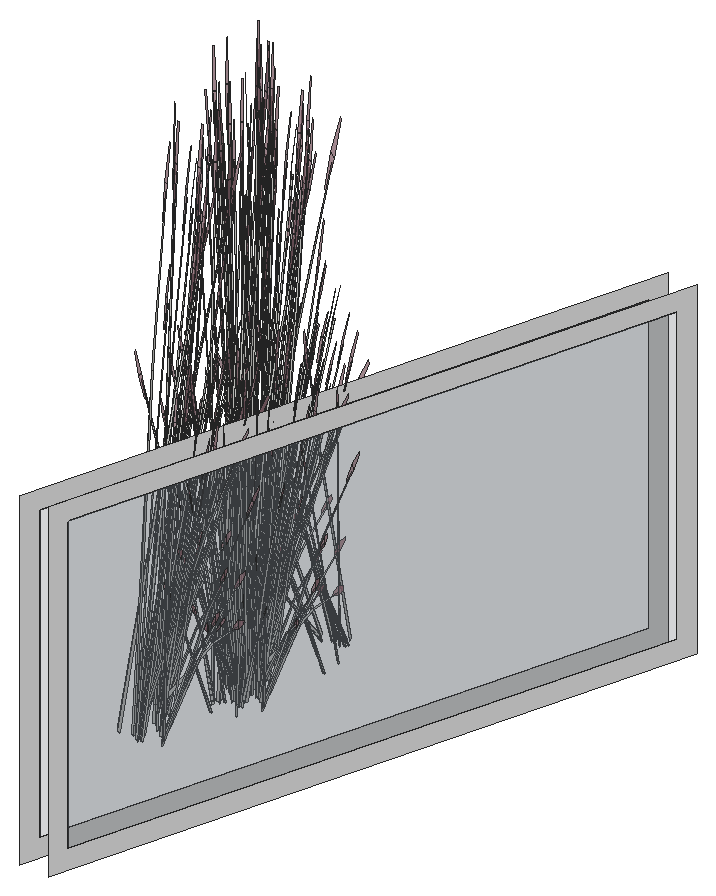
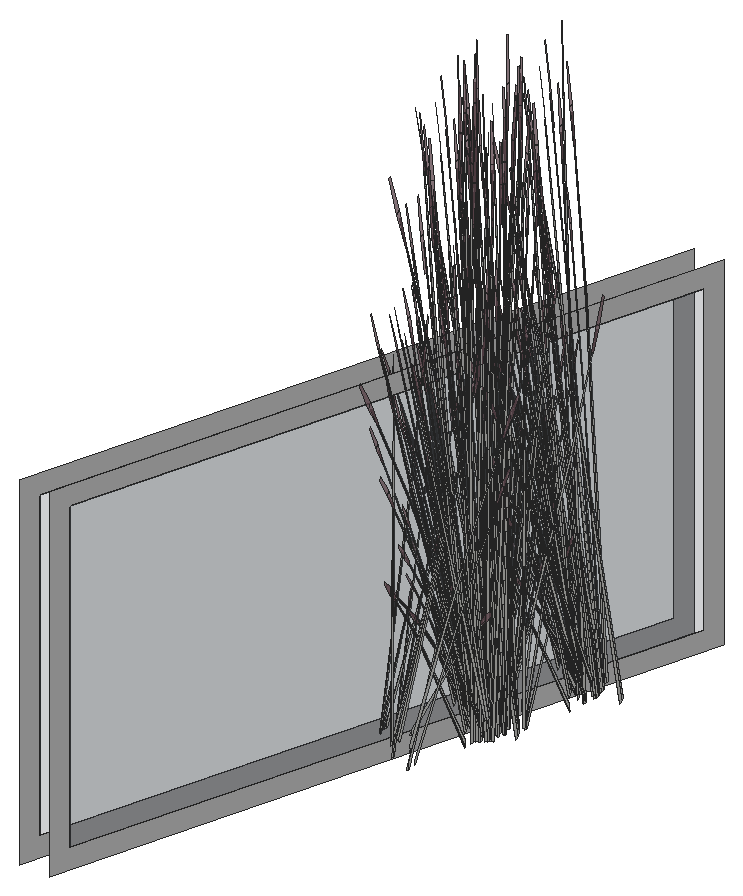
# SketchUp Ruby script. Lengths in inches.
U = 1.inch
M = Sketchup.active_model
def pt(a) = Geom::Point3d.new(a.map { |v| v * U })
def face(e, loops, mat)
  f = e.add_face(loops[0].map { |a| pt(a) })
  loops[1..].each { |l| e.add_face(l.map { |a| pt(a) }).erase! }
  f.material = f.back_material = mat if mat
  f
end
# faces: each face lists its corners as indices into pts; further lists are holes
def faces(e, pts, list, mat = nil) = list.each { |f| face(e, (f[0].is_a?(Array) ? f : [f]).map { |l| l.map { |i| pts[i] } }, mat) }
# xy, xz, yz: faces in a plane at the given z, y or x. An outline is a flat list of corners, or four numbers for a rectangle; further outlines are holes
def ring(l) = l.size == 4 ? [[l[0], l[1]], [l[2], l[1]], [l[2], l[3]], [l[0], l[3]]] : l.each_slice(2).to_a
def flat(e, list, mat, &to3) = list.each { |f| face(e, (f[0].is_a?(Array) ? f : [f]).map { |l| ring(l).map { |u, v| to3.(u, v) } }, mat) }
def xy(e, z, list, mat = nil) = flat(e, list, mat) { |x, y| [x, y, z] }
def xz(e, y, list, mat = nil) = flat(e, list, mat) { |x, z| [x, y, z] }
def yz(e, x, list, mat = nil) = flat(e, list, mat) { |y, z| [x, y, z] }
def lines(e, pts, list) = list.each { |a, b| e.add_line(pt(pts[a]), pt(pts[b])) }
# prism: a flat outline (further loops are holes) pulled along v
def prism(e, loops, v, mat = nil)
  f = face(e, loops, mat); d = Geom::Vector3d.new(v.map { |x| x * U })
  f.pushpull(f.normal.samedirection?(d) ? d.length : -d.length)
end
def box(e, o, s, mat = nil) = prism(e, [[o, [o[0] + s[0], o[1], o[2]], [o[0] + s[0], o[1] + s[1], o[2]], [o[0], o[1] + s[1], o[2]]]], [0, 0, s[2]], mat)
def at(x, y, z, deg = 0) = Geom::Transformation.translation(pt([x, y, z])) * Geom::Transformation.rotation(ORIGIN, Z_AXIS, deg.degrees)
def axes(o, x, y, z) = Geom::Transformation.new([*x, 0, *y, 0, *z, 0, *pt(o).to_a, 1])
def part(name) = M.definitions.add(name)
# library, detail: a bought-in or finely detailed component or shape, given as its bounding box
def library(name, o, s) = part(name).tap { |d| box(d.entities, o, s) }
def detail(e, o, s) = box(e.add_group.entities, o, s)
def put(e, d, t, mat = nil) = e.add_instance(d, t).tap { |i| i.material = mat if mat }
def group(e, t, mat = nil) = e.add_group.tap { |g| g.transformation = t; g.material = mat if mat }.entities
root = M.entities
M.materials.add("Glass_Basic_01").color = [105, 113, 122]
M.materials["Glass_Basic_01"].alpha = 0.25
M.materials.add("LightPink_Translucent").color = [144, 107, 117]
M.materials["LightPink_Translucent"].alpha = 0.75
M.materials.add("M01_Silver_Fog").color = [224, 224, 224]
c1 = part("blade")
p = [[2.15,0.21,22],[0,0.17,0],[0.09,0.45,0],[2.18,0.31,22],[2.29,0.31,22],[0.38,0.45,0],
  [2.48,0.24,33],[2.49,0.24,33],[2.48,0.22,33]]
faces(c1.entities,p,[[0,1,2,3],[4,5,2,3],[6,3,4,7],[8,0,3,6]])
c2 = part("seeds")
p = [[0.3,-0.1,1.38],[-0.01,-0.03,1.59],[-0.01,-0.03,0.03],[0.14,-0.07,-0.07],[0.29,-0.03,3],[0.15,0.01,3.11]]
faces(c2.entities,p,[[0,1,2,3],[1,0,4,5]],"LightPink_Translucent")
c3 = part("blade with seeds")
put(c3.entities,c1,at(0,0,0))
put(c3.entities,c2,axes([2.4,0.25,30.99],[1.5799,-0.05474,1.17369],[-0.12525,1.92788,0.29478],[-0.07173,-0.02425,1.56792]))
p = [[321.22,307.35,306],[340.07,371.78,306],[340.07,371.78,270],[321.22,307.35,270],[339.51,369.86,272],[339.51,369.86,304],
  [321.78,309.27,304],[321.78,309.27,272],[343.2,371.78,306],[324.34,307.35,306],[324.34,307.35,270],[343.2,371.78,270],
  [324.9,309.27,272],[324.9,309.27,304],[342.64,369.86,304],[342.64,369.86,272]]
faces(root,p,[[[0,1,2,3],[4,5,6,7]],[[8,9,10,11],[12,13,14,15]]],"M01_Silver_Fog")
faces(root,p,[[5,4,7,6],[13,12,15,14]],"Glass_Basic_01")
put(root,c3,axes([321.23,333.72,274.13],[-0.34721,0.30895,-0.03893],[-0.31814,-0.33837,-0.17649],[-0.0224,-0.09588,0.58215]))
put(root,c3,axes([321.09,336.77,274.36],[0.63506,0.11347,0.45755],[-0.12924,0.64083,0.17955],[-0.09281,-0.06188,1.58856]))
put(root,c3,axes([319.37,326.4,274.67],[0.56585,0.25696,-0.29095],[-0.27246,0.54236,-0.50002],[0.01778,0.13316,1.59708]))
put(root,c3,axes([320.92,336.65,274.72],[-0.24378,0.48527,0.44739],[-0.50654,-0.23354,-0.21531],[0,-0.11186,1.43643]))
put(root,c3,axes([321.73,334.32,276.98],[-0.23981,-0.43789,-0.71045],[0.49365,-0.24404,0.08574],[-0.05608,-0.21158,1.00501]))
put(root,c3,axes([320.75,337.79,274.47],[0.53992,-0.14294,0.17642],[0.13332,0.53195,0.35086],[-0.04815,-0.07751,1.60407]))
put(root,c3,axes([320.6,326.53,274.48],[0,-0.53854,0.49651],[0.56215,0,0],[0,0.12266,1.57504]))
put(root,c3,axes([320.84,327.03,274.02],[0,0.53854,-0.49651],[-0.56215,0,0],[0,0.12266,1.57504]))
put(root,c3,axes([319.34,328.66,276.73],[-0.49974,0.12359,0.48003],[-0.08673,-0.48481,0.3958],[0.11753,0.14288,0.9933]))
put(root,c3,axes([319.24,328.75,276.73],[-0.22836,0.34211,0.0643],[-0.3252,-0.19918,0.50621],[0.10513,0.10968,0.77189]))
put(root,c3,axes([321.44,337.88,274.2],[-0.50654,-0.24178,0],[0.24378,-0.50239,0],[0,0,1.62707]))
put(root,c3,axes([321.82,334.38,277.05],[-0.15148,0.41415,0.35414],[-0.44193,-0.12079,-0.4572],[-0.04052,-0.16674,0.87481]))
put(root,c3,axes([318.66,327.625,275.875],[-0.11485,-0.17291,1.71376],[0.53072,-0.14557,0.13857],[0.11995,0.27145,0.73262]))
put(root,c3,axes([322.61,338.48,274.375],[0.31414,0.53965,0],[-0.52557,0.30095,-0.51607],[-0.1197,0.06854,1.63711]))
put(root,c3,axes([319,325.68,274.62],[0.09693,-0.48062,0.1448],[0.47357,0.08343,-0.41347],[0.08619,0.04935,1.26744]))
put(root,c3,axes([321.02,338.72,277.0625],[-0.4951,-0.14079,0.53283],[0.1693,-0.46287,0.43934],[0.02975,0.18203,1.10256]))
put(root,c3,axes([320.88,338.75,276.73],[-0.37023,0.18303,0.0643],[-0.18122,-0.33376,0.50621],[0.03575,0.14712,0.77189]))
put(root,c3,axes([319.67,324.84,274.48],[-0.47024,-0.26927,0.49651],[0.28107,-0.48284,0],[0.1071,0.06133,1.57504]))
put(root,c3,axes([322.35,337.82,274.47],[0.14515,-0.53522,0.17642],[0.53115,0.15146,0.35086],[-0.09175,0.00261,1.60407]))
put(root,c3,axes([322.11,337.11,274.62],[0.37121,0.32357,0.1448],[-0.30963,0.36505,-0.41347],[-0.08619,0.04935,1.26744]))
put(root,c3,axes([321.98,336.71,274.3],[-0.46736,-0.46353,-0.06131],[0.46764,-0.46381,0],[-0.01632,-0.01619,1.75571]))
put(root,c3,axes([319.26,327.66,274.18],[0.5275,-0.18273,-0.19198],[0.18536,0.52636,0.00008],[0.05823,-0.0202,1.73897]))
put(root,c3,axes([322.1,336.875,274.72],[0.54562,-0.03324,0.44739],[0.04934,0.55185,-0.21531],[-0.09768,0.05593,1.43643]))
put(root,c3,axes([322.23,338.15,274.33],[0.62903,0.17504,0.30756],[-0.15737,0.62568,-0.36492],[-0.10411,0.07831,1.64885]))
put(root,c3,axes([321.31,333.35,273.49],[-0.08428,0.0194,1.76342],[-0.46606,-0.21841,-0.26939],[0.00782,-0.18218,0.30037]))
put(root,c3,axes([322.5,338.11,274.48],[0.47024,-0.26927,0.49651],[0.28107,0.48284,0],[-0.1071,0.06133,1.57504]))
put(root,c3,axes([319.17,328.36,277.05],[-0.0776,-0.43378,0.35414],[0.44361,-0.11454,-0.4572],[0.11915,0.12431,0.87481]))
put(root,c3,axes([321.77,333.94,276.53],[0.15148,-0.41415,-0.35414],[0.44193,0.12079,0.4572],[-0.04052,-0.16674,0.87481]))
put(root,c3,axes([321.03,336.18,274.36],[0.21845,0.6022,0.45755],[-0.62418,0.20941,0.17955],[0.00763,-0.11065,1.58856]))
put(root,c3,axes([319.27,326.09,274.21],[0.30184,0.45202,-0.44739],[-0.45719,0.31831,0.21531],[0.09768,0.05593,1.43643]))
put(root,c3,axes([320.93,336.1,274.21],[0.24378,-0.48527,-0.44739],[0.50654,0.23354,0.21531],[0,-0.11186,1.43643]))
put(root,c3,axes([321.56,337.67,274.2],[-0.16394,-0.4643,0],[0.46814,-0.1626,0],[0,0,1.54371]))
put(root,c3,axes([323.47,345,274.59],[-0.03043,0.17617,1.43002],[-0.4448,0.14748,-0.30754],[-0.10397,-0.22771,0.61141]))
put(root,c3,axes([319.47,325.87,276.47],[-0.43417,-0.27982,1.38283],[0.45844,-0.43566,0.59665],[0.14008,0.26255,1.33663]))
put(root,c3,axes([323.61,345.46,275.875],[0.11485,0.17291,1.71376],[-0.53072,0.14557,0.13857],[-0.11995,-0.27145,0.73262]))
put(root,c3,axes([318.74,328.97,276.71],[0.00149,-0.0652,1.77383],[0.43058,-0.28766,-0.16761],[0.14956,0.10267,0.31391]))
put(root,c3,axes([320.125,328.14,274.77],[-0.2829,-0.15485,1.1486],[0.36529,-0.15734,0.84392],[0.09853,0.13328,0.25299]))
put(root,c3,axes([319.12,327.98,274.59],[0.00887,-0.17852,1.43002],[0.42372,-0.19941,-0.30754],[0.1308,0.21367,0.61141]))
put(root,c3,axes([322.22,336.75,274.21],[-0.24378,0.48527,-0.44739],[-0.50654,-0.23354,0.21531],[0,0.11186,1.43643]))
put(root,c3,axes([320.1,325.09,274.03],[0.11803,0.46926,-0.30978],[-0.46876,0.13325,0.30978],[0.0945,0.05411,1.38974]))
put(root,c3,axes([321.96,334.01,276.73],[0.37023,-0.18303,0.0643],[0.18122,0.33376,0.50621],[-0.03575,-0.14712,0.77189]))
put(root,c3,axes([320.98,326.62,274.375],[0.62828,0,0],[0,0.6019,-0.51607],[0,0.13709,1.63711]))
put(root,c3,axes([323.18,336.46,274.47],[-0.39477,-0.39228,0.17642],[0.39783,-0.38049,0.35086],[-0.0436,0.08011,1.60407]))
put(root,c3,axes([321.82,336.23,274.21],[0,-0.62313,0],[0.62828,0,0],[0,0,1.79456]))
put(root,c3,axes([321.83,334.04,276.73],[0.4951,0.14079,0.48003],[-0.1693,0.46287,0.3958],[-0.02975,-0.18203,0.9933]))
put(root,c3,axes([321.24,336.35,274.43],[0.56613,0.26102,0.24065],[-0.27246,0.54236,0.50002],[0,-0.12502,1.60543]))
put(root,c3,axes([322.14,336.48,274.29],[0,0.62282,-0.05637],[-0.62828,0,0],[0,0.01957,1.79368]))
put(root,c3,axes([318.95,325.84,274.67],[0.5073,-0.35754,-0.29095],[0.33735,0.5052,-0.50002],[0.12516,0.05131,1.59708]))
put(root,c3,axes([321.05,335.98,274.72],[-0.54562,0.03324,0.44739],[-0.04934,-0.55185,-0.21531],[0.09768,-0.05593,1.43643]))
put(root,c3,axes([320.17,328.85,274.67],[-0.3222,-0.01689,1.0506],[0.21278,-0.35872,0.58006],[0.12729,0.12745,0.8241]))
put(root,c3,axes([321.02,338.375,277.05],[0.15148,-0.41415,0.35414],[0.44193,0.12079,-0.4572],[0.04052,0.16674,0.87481]))
put(root,c3,axes([320.8,335.03,274.47],[-0.14515,0.53522,0.17642],[-0.53115,-0.15146,0.35086],[0.09175,-0.00261,1.60407]))
put(root,c3,axes([321.83,337.69,274.29],[0.21845,0.61869,-0.06012],[-0.62418,0.21679,0],[0.00763,0.02161,1.72173]))
put(root,c3,axes([320.54,334.375,274.375],[-0.31414,-0.53965,0],[0.52557,-0.30095,-0.51607],[0.1197,-0.06854,1.63711]))
put(root,c3,axes([323.64,336.875,274.2],[-0.62797,-0.00431,-0.04976],[0,-0.6019,0.49943],[-0.01973,0.13702,1.58352]))
put(root,c3,axes([319.13,328.59,277.03],[0.2994,-0.46097,-0.1216],[0.43359,0.26557,-0.67495],[0.15072,0.13024,1.02557]))
put(root,c3,axes([317.67,325.52,273.59],[-0.49456,0.21561,1.28929],[-0.15741,-0.61865,0.50096],[0.30369,0.01029,1.46642]))
put(root,c3,axes([322.41,335.0625,274.47],[-0.53992,0.14294,0.17642],[-0.13332,-0.53195,0.35086],[0.04815,0.07751,1.60407]))
put(root,c3,axes([321.85,333.07,274.77],[0.06446,0.31404,1.1486],[-0.35756,-0.17393,0.84392],[0.03848,-0.1608,0.25299]))
put(root,c3,axes([321.62,339.85,277.65],[0.34721,-0.30895,-0.06488],[0.31814,0.33837,-0.29416],[0.0224,0.09588,0.97024]))
put(root,c3,axes([319.49,328.36,276.68],[0.4958,-0.12802,-0.51099],[0.08673,0.48481,-0.3958],[0.13317,0.13893,0.97773]))
put(root,c3,axes([321.52,335.84,274.36],[-0.4166,0.48873,0.45755],[-0.49494,-0.43142,0.17955],[0.10044,-0.04877,1.58856]))
put(root,c3,axes([322.23,336.61,274.21],[0.35073,0.34786,0],[-0.35073,0.34786,0],[0,0,1.69266]))
put(root,c3,axes([319.94,324.5625,274.375],[0.31414,-0.53965,0],[0.52557,0.30095,-0.51607],[0.1197,0.06854,1.63711]))
put(root,c3,axes([322.23,336.2,274.72],[0.24378,-0.48527,0.44739],[0.50654,0.23354,-0.21531],[0,0.11186,1.43643]))
put(root,c3,axes([322.02,337.89,274.2],[0.50654,0.24178,0],[-0.24378,0.50239,0],[0,0,1.74954]))
put(root,c3,axes([320.05,327.77,277.05],[-0.28589,-0.33718,0.35414],[0.32644,-0.31919,-0.4572],[0.16586,0.04856,0.87481]))
put(root,c3,axes([320.23,324.89,274.02],[0.47024,0.26927,-0.49651],[-0.28107,0.48284,0],[0.1071,0.06133,1.57504]))
put(root,c3,axes([324.49,344.3125,276.72],[-0.07685,-0.07551,1.74944],[-0.51287,0.04787,-0.27667],[-0.08185,-0.1806,0.14031]))
put(root,c3,axes([320.875,338.55,277.03],[0.49168,-0.25073,-0.1216],[0.24162,0.44501,-0.67495],[0.06487,0.18753,1.02557]))
put(root,c3,axes([320.3125,328.08,276.73],[-0.0253,0.40952,0.0643],[-0.38204,-0.01123,0.50621],[0.14634,0.04285,0.77189]))
put(root,c3,axes([322.0625,336.09,274.38],[-0.63506,-0.11347,0.49198],[0.12924,-0.64083,0.19306],[0.09281,0.06188,1.70813]))
put(root,c3,axes([323.39,333.58,276.71],[-0.05103,0.04113,1.77383],[-0.49994,-0.13878,-0.16761],[-0.0181,-0.17951,0.31391]))
put(root,c3,axes([320.2,328.72,273.49],[0.03661,-0.07775,1.76342],[0.46087,-0.22898,-0.26939],[0.13972,0.11851,0.30037]))
put(root,c3,axes([322.99,334.77,277.03],[-0.55221,-0.02668,-0.1216],[0.01509,-0.50521,-0.67495],[0.03836,-0.19458,1.02557]))
put(root,c3,axes([320.35,327.95,276.73],[-0.37048,0.35486,0.48003],[-0.31952,-0.37685,0.3958],[0.17382,0.06546,0.9933]))
put(root,c3,axes([323.51,336.96,274.03],[-0.35073,0.33601,-0.30978],[-0.35073,-0.33601,0.30978],[0,0.10823,1.38974]))
put(root,c3,axes([321.3125,328,275.93],[-0.09617,-0.45271,-0.03492],[0.45453,-0.10408,-0.15832],[0.09492,0.0287,0.52218]))
put(root,c3,axes([320.52,326.83,277.05],[-0.41757,-0.15024,0.35414],[0.12179,-0.4383,-0.4572],[0.16812,-0.04019,0.87481]))
put(root,c3,axes([322.51,336.9,274.09],[0.18424,0.49308,-0.69212],[-0.53071,0.17758,-0.18165],[0.02036,0.16697,1.52773]))
put(root,c3,axes([322.25,336.37,274.21],[0.56215,0,0],[0,0.55754,0],[0,0,1.78407]))
put(root,c3,axes([319.54,325.92,274.06],[0.52267,0.08829,-0.62353],[-0.11029,0.54463,-0.16365],[0.15598,0.06599,1.37633]))
put(root,c3,axes([322.78,334.85,277.05],[-0.33997,0.28354,0.35414],[-0.32182,-0.32376,-0.4572],[0.04897,-0.1645,0.87481]))
put(root,c3,axes([321.71,335.76,274.72],[-0.30184,-0.45202,0.44739],[0.45719,-0.31831,-0.21531],[0.09768,0.05593,1.43643]))
put(root,c3,axes([321.77,326.24,274.26],[-0.31151,-0.34437,-0.06488],[0.34117,-0.31553,-0.29416],[0.09667,-0.02221,0.97024]))
put(root,c3,axes([321.16,335.86,274.67],[-0.05855,-0.61451,-0.29095],[0.60981,-0.03716,-0.50002],[0.10738,-0.08185,1.59708]))
put(root,c3,axes([322.44,336.3125,274.62],[0.46814,-0.15705,0.1448],[0.16394,0.44848,-0.41347],[0,0.0987,1.26744]))
put(root,c3,axes([322.62,334.58,276.68],[-0.35968,-0.36185,-0.51099],[0.37996,-0.3169,-0.3958],[0.05473,-0.18385,0.97773]))
put(root,c3,axes([324.85,345.5,276.68],[-0.49392,-0.135,-0.51099],[0.1693,-0.46287,-0.3958],[-0.04529,-0.18636,0.97773]))
put(root,c3,axes([322.28,336.35,274.67],[0.56585,0.25696,-0.29095],[-0.27246,0.54236,-0.50002],[0.01778,0.13316,1.59708]))
put(root,c3,axes([321.08,334.5,274.03],[0.46876,0.13325,-0.30978],[-0.11803,0.46926,0.30978],[0.0945,-0.05411,1.38974]))
put(root,c3,axes([322.38,333.9375,274.59],[-0.14282,0.10901,1.43002],[-0.42773,-0.19079,-0.30754],[0.07929,-0.23728,0.61141]))
put(root,c3,axes([319.43,327.09,275.875],[-0.18664,-0.09279,1.71376],[0.38624,-0.38925,0.13857],[0.24072,0.1756,0.73262]))
put(root,c3,axes([323.51,336.47,274.48],[0,-0.53854,0.49651],[0.56215,0,0],[0,0.12266,1.57504]))
put(root,c3,axes([323.75,336.97,274.02],[0,0.53854,-0.49651],[-0.56215,0,0],[0,0.12266,1.57504]))
put(root,c3,axes([322.25,338.6,276.73],[-0.49974,0.12359,0.48003],[-0.08673,-0.48481,0.3958],[0.11753,0.14288,0.9933]))
put(root,c3,axes([320.97,334.29,274.02],[0.47024,-0.26927,-0.49651],[0.28107,0.48284,0],[0.1071,-0.06133,1.57504]))
put(root,c3,axes([322.15,338.7,276.73],[-0.22836,0.34211,0.0643],[-0.3252,-0.19918,0.50621],[0.10513,0.10968,0.77189]))
put(root,c3,axes([321.91,335.63,274.62],[0.09693,-0.48062,0.1448],[0.47357,0.08343,-0.41347],[0.08619,0.04935,1.26744]))
put(root,c3,axes([325.03,345.59,276.98],[-0.23981,-0.43789,-0.71045],[0.49365,-0.24404,0.08574],[-0.05608,-0.21158,1.00501]))
put(root,c3,axes([320.9,326.97,276.73],[0.18454,0.3672,0.0643],[-0.33652,0.17973,0.50621],[0.14834,-0.03546,0.77189]))
put(root,c3,axes([320.46,327.95,276.53],[0.28589,0.33718,-0.35414],[-0.32644,0.31919,0.4572],[0.16586,0.04856,0.87481]))
put(root,c3,axes([320.13,327.99,277.03],[0.0269,-0.54769,-0.1216],[0.50939,0.01497,-0.67495],[0.19618,0.03804,1.02557]))
put(root,c3,axes([320.7,326.98,277.03],[-0.25281,-0.48765,-0.1216],[0.44869,-0.23964,-0.67495],[0.18908,-0.06434,1.02557]))
put(root,c3,axes([320.87,326.84,276.73],[-0.14195,0.49104,0.48003],[-0.46669,-0.16791,0.3958],[0.18353,-0.02951,0.9933]))
put(root,c3,axes([322.58,334.79,274.48],[-0.47024,-0.26927,0.49651],[0.28107,-0.48284,0],[0.1071,0.06133,1.57504]))
put(root,c3,axes([322.73,334.74,276.98],[0.01307,-0.49815,-0.71045],[0.55054,0.03346,0.08574],[0.0581,-0.21104,1.00501]))
put(root,c3,axes([322.17,337.6,274.18],[0.5275,-0.18273,-0.19198],[0.18536,0.52636,0.00008],[0.05823,-0.0202,1.73897]))
put(root,c3,axes([322.08,338.31,277.05],[-0.0776,-0.43378,0.35414],[0.44361,-0.11454,-0.4572],[0.11915,0.12431,0.87481]))
put(root,c3,axes([320.58,327.66,276.72],[0.10779,-0.00911,1.74944],[0.29564,-0.41839,-0.27667],[0.19172,0.05523,0.14031]))
put(root,c3,axes([322.18,336.04,274.21],[0.30184,0.45202,-0.44739],[-0.45719,0.31831,0.21531],[0.09768,0.05593,1.43643]))
put(root,c3,axes([320.68,326.56,276.68],[0.13612,-0.48987,-0.51099],[0.46669,0.16791,-0.3958],[0.1879,-0.04492,0.97773]))
put(root,c3,axes([322.38,335.8125,276.47],[-0.43417,-0.27982,1.38283],[0.45844,-0.43566,0.59665],[0.14008,0.26255,1.33663]))
put(root,c3,axes([322.95,334.45,276.53],[0.33997,-0.28354,-0.35414],[0.32182,0.32376,0.4572],[0.04897,-0.1645,0.87481]))
put(root,c3,axes([321.85,326.87,274.77],[-0.31044,0.08891,1.1486],[0.14613,-0.36744,0.84392],[0.16469,0.02514,0.25299]))
put(root,c3,axes([321.65,338.91,276.71],[0.00149,-0.0652,1.77383],[0.43058,-0.28766,-0.16761],[0.14956,0.10267,0.31391]))
put(root,c3,axes([323.08,334.59,276.73],[0.4129,0.02509,0.0643],[-0.01132,0.37891,0.50621],[0.04321,-0.14514,0.77189]))
put(root,c3,axes([323.04,338.09,274.77],[-0.2829,-0.15485,1.1486],[0.36529,-0.15734,0.84392],[0.09853,0.13328,0.25299]))
put(root,c3,axes([322.03,337.93,274.59],[0.00887,-0.17852,1.43002],[0.42372,-0.19941,-0.30754],[0.1308,0.21367,0.61141]))
put(root,c3,axes([324.61,344.62,273.49],[-0.08428,0.0194,1.76342],[-0.46606,-0.21841,-0.26939],[0.00782,-0.18218,0.30037]))
put(root,c3,axes([323.49,333.97,276.72],[-0.00485,-0.10718,1.74944],[-0.40965,-0.30977,-0.27667],[0.06333,-0.18778,0.14031]))
put(root,c3,axes([321.52,335.39,274.06],[0.33843,-0.40479,-0.62353],[0.42041,0.36705,-0.16365],[0.13561,-0.10098,1.37633]))
put(root,c3,axes([322.95,334.56,276.73],[0.35779,0.36745,0.48003],[-0.37996,0.3169,0.3958],[0.066,-0.17239,0.9933]))
put(root,c3,axes([320.96,326.78,276.53],[0.41757,0.15024,-0.35414],[-0.12179,0.4383,0.4572],[0.16812,-0.04019,0.87481]))
put(root,c3,axes([325.07,345.22,276.53],[0.15148,-0.41415,-0.35414],[0.44193,0.12079,0.4572],[-0.04052,-0.16674,0.87481]))
put(root,c3,axes([320.16,327.73,276.98],[0.50227,0.01297,-0.71045],[-0.03373,0.54602,0.08574],[0.21278,0.05762,1.00501]))
put(root,c3,axes([323.01,335.04,274.03],[0.11803,0.46926,-0.30978],[-0.46876,0.13325,0.30978],[0.0945,0.05411,1.38974]))
put(root,c3,axes([323.89,336.56,274.375],[0.62828,0,0],[0,0.6019,-0.51607],[0,0.13709,1.63711]))
put(root,c3,axes([321.18,326.7,273.98],[-0.32361,0.06463,1.41583],[-0.05151,-0.51444,0.08104],[0.22666,-0.07786,0.80566]))
put(root,c3,axes([321.53,326.36,273.49],[-0.02626,-0.08176,1.76342],[0.18213,-0.47826,-0.26939],[0.18372,-0.00688,0.30037]))
put(root,c3,axes([321.71,328.42,276.71],[-0.04543,-0.04715,1.77383],[0.09938,-0.50538,-0.16761],[0.17896,-0.03229,0.31391]))
put(root,c3,axes([321.86,335.78,274.67],[0.5073,-0.35754,-0.29095],[0.33735,0.5052,-0.50002],[0.12516,0.05131,1.59708]))
put(root,c3,axes([319.83,326.24,275.875],[-0.20841,0.0122,1.71376],[0.13825,-0.52864,0.13857],[0.297,0.0327,0.73262]))
put(root,c3,axes([323.08,338.8,274.67],[-0.3222,-0.01689,1.0506],[0.21278,-0.35872,0.58006],[0.12729,0.12745,0.8241]))
put(root,c3,axes([323.37,335.72,277.05],[-0.43736,0.07697,0.35414],[-0.11549,-0.43998,-0.4572],[0.12533,-0.11818,0.87481]))
put(root,c3,axes([322.11,334.49,275.875],[-0.09355,0.18511,1.71376],[-0.39247,-0.38307,0.13857],[0.17705,-0.23875,0.73262]))
put(root,c3,axes([320.59,326.74,276.98],[0.44151,-0.23785,-0.71045],[0.24605,0.4896,0.08574],[0.21333,-0.05562,1.00501]))
put(root,c3,axes([322.04,338.53,277.03],[0.2994,-0.46097,-0.1216],[0.43359,0.26557,-0.67495],[0.15072,0.13024,1.02557]))
put(root,c3,axes([320.58,335.47,273.59],[-0.49456,0.21561,1.28929],[-0.15741,-0.61865,0.50096],[0.30369,0.01029,1.46642]))
put(root,c3,axes([323.59,335.76,277.03],[-0.46478,-0.29695,-0.1216],[0.26776,-0.43004,-0.67495],[0.13131,-0.14949,1.02557]))
put(root,c3,axes([322.4,338.3,276.68],[0.4958,-0.12802,-0.51099],[0.08673,0.48481,-0.3958],[0.13317,0.13893,0.97773]))
put(root,c3,axes([321.27,327.46,274.59],[-0.12101,-0.13245,1.43002],[0.15744,-0.43816,-0.30754],[0.24483,0.05936,0.61141]))
put(root,c3,axes([322.85,334.51,274.375],[0.31414,-0.53965,0],[0.52557,0.30095,-0.51607],[0.1197,0.06854,1.63711]))
put(root,c3,axes([323.38,334.27,273.49],[-0.0752,-0.04243,1.76342],[-0.19317,-0.47398,-0.26939],[0.13031,-0.12863,0.30037]))
put(root,c3,axes([322.97,337.72,277.05],[-0.28589,-0.33718,0.35414],[0.32644,-0.31919,-0.4572],[0.16586,0.04856,0.87481]))
put(root,c3,axes([323.14,334.83,274.02],[0.47024,0.26927,-0.49651],[-0.28107,0.48284,0],[0.1071,0.06133,1.57504]))
put(root,c3,axes([323.23,338.03,276.73],[-0.0253,0.40952,0.0643],[-0.38204,-0.01123,0.50621],[0.14634,0.04285,0.77189]))
put(root,c3,axes([323.11,338.67,273.49],[0.03661,-0.07775,1.76342],[0.46087,-0.22898,-0.26939],[0.13972,0.11851,0.30037]))
put(root,c3,axes([323.26,337.9,276.73],[-0.37048,0.35486,0.48003],[-0.31952,-0.37685,0.3958],[0.17382,0.06546,0.9933]))
put(root,c3,axes([323.36,335.41,276.68],[-0.12908,-0.49174,-0.51099],[0.48882,-0.08602,-0.3958],[0.14008,-0.13208,0.97773]))
put(root,c3,axes([324.22,337.95,275.93],[-0.09617,-0.45271,-0.03492],[0.45453,-0.10408,-0.15832],[0.09492,0.0287,0.52218]))
put(root,c3,axes([323.4375,336.78,277.05],[-0.41757,-0.15024,0.35414],[0.12179,-0.4383,-0.4572],[0.16812,-0.04019,0.87481]))
put(root,c3,axes([322.45,335.87,274.06],[0.52267,0.08829,-0.62353],[-0.11029,0.54463,-0.16365],[0.15598,0.06599,1.37633]))
put(root,c3,axes([324.68,336.1875,274.26],[-0.31151,-0.34437,-0.06488],[0.34117,-0.31553,-0.29416],[0.09667,-0.02221,0.97024]))
put(root,c3,axes([326.68,344.85,276.71],[-0.05103,0.04113,1.77383],[-0.49994,-0.13878,-0.16761],[-0.0181,-0.17951,0.31391]))
put(root,c3,axes([323.96,334.43,274.77],[-0.16736,0.27414,1.1486],[-0.14385,-0.36832,0.84392],[0.13822,-0.09229,0.25299]))
put(root,c3,axes([323.76,335.65,276.73],[0.34493,0.22649,0.0643],[-0.20082,0.32253,0.50621],[0.11059,-0.10427,0.77189]))
put(root,c3,axes([323.67,335.56,276.73],[0.12461,0.49565,0.48003],[-0.48882,0.08602,0.3958],[0.14406,-0.11657,0.9933]))
put(root,c3,axes([322.34,337.03,275.875],[-0.18664,-0.09279,1.71376],[0.38624,-0.38925,0.13857],[0.24072,0.1756,0.73262]))
put(root,c3,axes([324.74,335.64,276.71],[-0.06563,-0.00409,1.77383],[-0.27252,-0.43825,-0.16761],[0.10944,-0.1441,0.31391]))
put(root,c3,axes([323.72,335.46,276.53],[0.43736,-0.07697,-0.35414],[0.11549,0.43998,0.4572],[0.12533,-0.11818,0.87481]))
put(root,c3,axes([323.375,335.61,276.98],[0.26246,-0.42493,-0.71045],[0.45991,0.30199,0.08574],[0.15671,-0.15395,1.00501]))
put(root,c3,axes([323.81,336.91,276.73],[0.18454,0.3672,0.0643],[-0.33652,0.17973,0.50621],[0.14834,-0.03546,0.77189]))
put(root,c3,axes([323.37,337.9,276.53],[0.28589,0.33718,-0.35414],[-0.32644,0.31919,0.4572],[0.16586,0.04856,0.87481]))
put(root,c3,axes([323.04,337.9375,277.03],[0.0269,-0.54769,-0.1216],[0.50939,0.01497,-0.67495],[0.19618,0.03804,1.02557]))
put(root,c3,axes([323.61,336.92,277.03],[-0.25281,-0.48765,-0.1216],[0.44869,-0.23964,-0.67495],[0.18908,-0.06434,1.02557]))
put(root,c3,axes([323.78,336.78,276.73],[-0.14195,0.49104,0.48003],[-0.46669,-0.16791,0.3958],[0.18353,-0.02951,0.9933]))
put(root,c3,axes([325.68,345.21,274.59],[-0.14282,0.10901,1.43002],[-0.42773,-0.19079,-0.30754],[0.07929,-0.23728,0.61141]))
put(root,c3,axes([323.49,337.61,276.72],[0.10779,-0.00911,1.74944],[0.29564,-0.41839,-0.27667],[0.19172,0.05523,0.14031]))
put(root,c3,axes([326.03,346.02,276.98],[0.01307,-0.49815,-0.71045],[0.55054,0.03346,0.08574],[0.0581,-0.21104,1.00501]))
put(root,c3,axes([323.59,336.5,276.68],[0.13612,-0.48987,-0.51099],[0.46669,0.16791,-0.3958],[0.1879,-0.04492,0.97773]))
put(root,c3,axes([324.76,336.82,274.77],[-0.31044,0.08891,1.1486],[0.14613,-0.36744,0.84392],[0.16469,0.02514,0.25299]))
put(root,c3,axes([323.76,335.22,274.59],[-0.1795,-0.01595,1.43002],[-0.18389,-0.42791,-0.30754],[0.22051,-0.12105,0.61141]))
put(root,c3,axes([323.875,336.73,276.53],[0.41757,0.15024,-0.35414],[-0.12179,0.4383,0.4572],[0.16812,-0.04019,0.87481]))
put(root,c3,axes([323.07,337.67,276.98],[0.50227,0.01297,-0.71045],[-0.03373,0.54602,0.08574],[0.21278,0.05762,1.00501]))
put(root,c3,axes([324.09,336.64,273.98],[-0.32361,0.06463,1.41583],[-0.05151,-0.51444,0.08104],[0.22666,-0.07786,0.80566]))
put(root,c3,axes([324.44,336.31,273.49],[-0.02626,-0.08176,1.76342],[0.18213,-0.47826,-0.26939],[0.18372,-0.00688,0.30037]))
put(root,c3,axes([324.62,338.37,276.71],[-0.04543,-0.04715,1.77383],[0.09938,-0.50538,-0.16761],[0.17896,-0.03229,0.31391]))
put(root,c3,axes([322.74,336.19,275.875],[-0.20841,0.0122,1.71376],[0.13825,-0.52864,0.13857],[0.297,0.0327,0.73262]))
put(root,c3,axes([326.79,345.24,276.72],[-0.00485,-0.10718,1.74944],[-0.40965,-0.30977,-0.27667],[0.06333,-0.18778,0.14031]))
put(root,c3,axes([323.5,336.68,276.98],[0.44151,-0.23785,-0.71045],[0.24605,0.4896,0.08574],[0.21333,-0.05562,1.00501]))
put(root,c3,axes([324.98,336.16,276.72],[0.06972,-0.08203,1.74944],[-0.08924,-0.50318,-0.27667],[0.17494,-0.0954,0.14031]))
put(root,c3,axes([325.41,345.76,275.875],[-0.09355,0.18511,1.71376],[-0.39247,-0.38307,0.13857],[0.17705,-0.23875,0.73262]))
put(root,c3,axes([324.18,337.41,274.59],[-0.12101,-0.13245,1.43002],[0.15744,-0.43816,-0.30754],[0.24483,0.05936,0.61141]))
